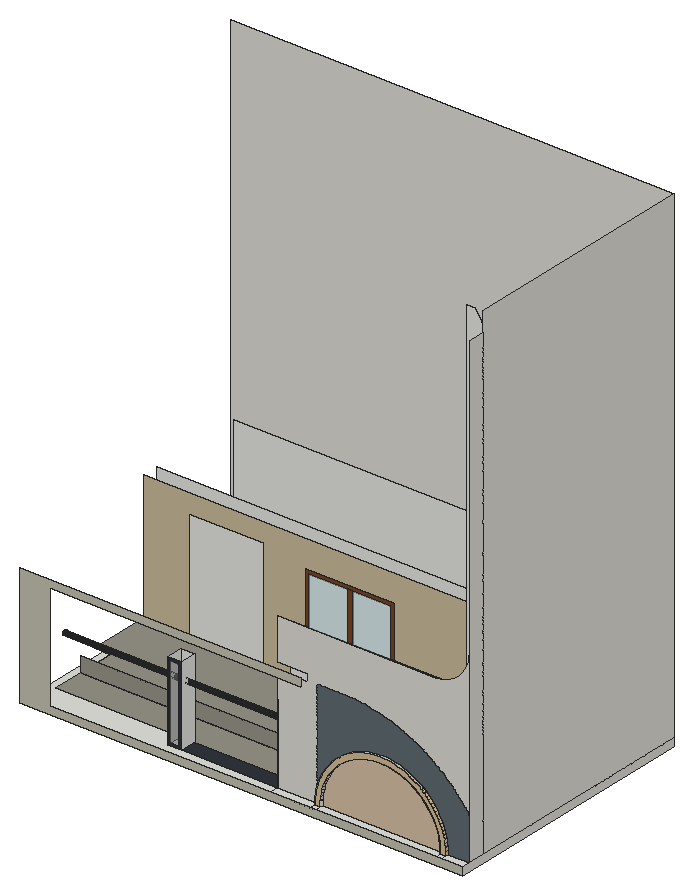
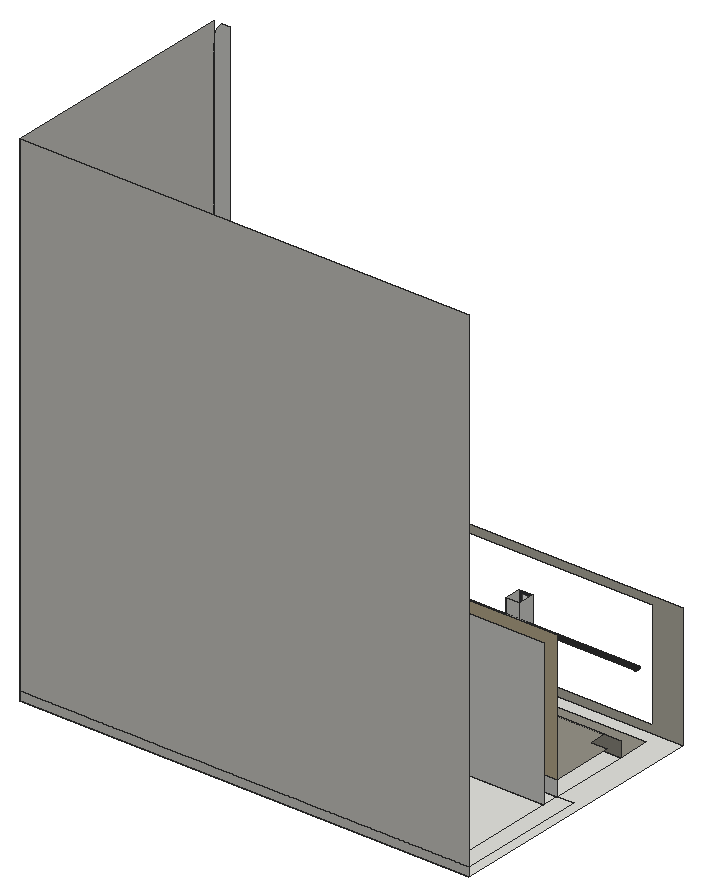
# SketchUp Ruby script. Lengths in inches.
U = 1.inch
M = Sketchup.active_model
def pt(a) = Geom::Point3d.new(a.map { |v| v * U })
def face(e, loops, mat)
  f = e.add_face(loops[0].map { |a| pt(a) })
  loops[1..].each { |l| e.add_face(l.map { |a| pt(a) }).erase! }
  f.material = f.back_material = mat if mat
  f
end
# faces: each face lists its corners as indices into pts; further lists are holes
def faces(e, pts, list, mat = nil) = list.each { |f| face(e, (f[0].is_a?(Array) ? f : [f]).map { |l| l.map { |i| pts[i] } }, mat) }
# xy, xz, yz: faces in a plane at the given z, y or x. An outline is a flat list of corners, or four numbers for a rectangle; further outlines are holes
def ring(l) = l.size == 4 ? [[l[0], l[1]], [l[2], l[1]], [l[2], l[3]], [l[0], l[3]]] : l.each_slice(2).to_a
def flat(e, list, mat, &to3) = list.each { |f| face(e, (f[0].is_a?(Array) ? f : [f]).map { |l| ring(l).map { |u, v| to3.(u, v) } }, mat) }
def xy(e, z, list, mat = nil) = flat(e, list, mat) { |x, y| [x, y, z] }
def xz(e, y, list, mat = nil) = flat(e, list, mat) { |x, z| [x, y, z] }
def yz(e, x, list, mat = nil) = flat(e, list, mat) { |y, z| [x, y, z] }
def lines(e, pts, list) = list.each { |a, b| e.add_line(pt(pts[a]), pt(pts[b])) }
# prism: a flat outline (further loops are holes) pulled along v
def prism(e, loops, v, mat = nil)
  f = face(e, loops, mat); d = Geom::Vector3d.new(v.map { |x| x * U })
  f.pushpull(f.normal.samedirection?(d) ? d.length : -d.length)
end
def box(e, o, s, mat = nil) = prism(e, [[o, [o[0] + s[0], o[1], o[2]], [o[0] + s[0], o[1] + s[1], o[2]], [o[0], o[1] + s[1], o[2]]]], [0, 0, s[2]], mat)
def at(x, y, z, deg = 0) = Geom::Transformation.translation(pt([x, y, z])) * Geom::Transformation.rotation(ORIGIN, Z_AXIS, deg.degrees)
def axes(o, x, y, z) = Geom::Transformation.new([*x, 0, *y, 0, *z, 0, *pt(o).to_a, 1])
def part(name) = M.definitions.add(name)
# library, detail: a bought-in or finely detailed component or shape, given as its bounding box
def library(name, o, s) = part(name).tap { |d| box(d.entities, o, s) }
def detail(e, o, s) = box(e.add_group.entities, o, s)
def put(e, d, t, mat = nil) = e.add_instance(d, t).tap { |i| i.material = mat if mat }
def group(e, t, mat = nil) = e.add_group.tap { |g| g.transformation = t; g.material = mat if mat }.entities
root = M.entities
M.materials.add("[Formica Beige]").color = [211, 187, 149]
M.materials.add("[Formica Graystone]").color = [193, 189, 175]
M.materials.add("[Formica Graystone]1").color = [149, 146, 135]
M.materials.add("[Formica Laminate Dark]").color = [50, 53, 60]
M.materials.add("[Formica Laminate Light]").color = [213, 189, 164]
M.materials.add("[Formica Speckled Grey]1").color = [94, 105, 111]
M.materials.add("[Quartz Light Brown]").color = [199, 184, 152]
M.materials.add("[Terrazzo Tile Light]").color = [219, 217, 210]
M.materials.add("[Translucent Glass Gray]").color = [128, 128, 128]
M.materials["[Translucent Glass Gray]"].alpha = 0.5
M.materials.add("[Translucent Glass Safety]").color = [204, 235, 244]
M.materials["[Translucent Glass Safety]"].alpha = 0.5
M.materials.add("[Wood Veneer 01]").color = [120, 70, 37]
xy(root,0,[[0,13.1875,490.375,305.18]])
xy(root,9,[[277.85,13.1875,321.38,22.75],[321.38,13.1875,327.45,19.625],[327.45,13.1875,460.44,22.75],[460.44,13.1875,466.51,19.625],[466.51,13.1875,490.375,22.75],
  [321.38,19.625,327.45,22.75],[460.44,19.625,466.51,22.75],[155.89,22.75,171.0625,40.6875],[277.85,22.75,490.375,40.6875],[472.4375,40.6875,490.375,162.27],
  [17.9375,75.25,472.4375,162.27],[0,162.27,0,305.18,490.375,305.18,490.375,162.27,472.4375,162.27,472.4375,287.24,17.9375,287.24,17.9375,162.27],[17.9375,162.27,472.4375,180.28],[17.9375,180.28,472.4375,287.24]])
xy(root,9,[[17.9375,40.6875,472.4375,75.25]],"[Formica Graystone]1")
xy(root,9,[[171.0625,22.75,277.85,40.6875]],"[Formica Laminate Dark]")
xy(root,25.4375,[[36.375,75.25,472.4375,75.25,472.4375,162.27,17.9375,162.27,17.9375,93.6875,36.375,93.6875]],"[Formica Graystone]1")
xz(root,13.1875,[[0,0,490.375,0,490.375,9,32.82,9,32.82,125.79,311.48,125.79,311.48,134.5,0,134.5]],"[Formica Graystone]")
xz(root,19.625,[[321.38,9,327.45,9,327.45,14.79,327.54,15.98,328,19.44,328.64,22.88,329.45,26.28,330.44,29.63,331.61,32.93,332.95,36.16,334.45,39.3125,336.12,42.38,337.95,45.36,339.93,48.25,342.06,51.02,344.33,53.68,346.73,56.21,349.27,58.62,351.93,60.89,354.7,63.02,357.58,65,360.5625,66.82,363.63,68.49,366.79,70,370.02,71.33,373.3125,72.5,376.66,73.49,380.0625,74.31,383.5,74.95,386.97,75.4,390.45,75.68,393.95,75.77,397.44,75.68,400.92,75.4,404.39,74.95,407.83,74.31,411.23,73.49,414.58,72.5,417.875,71.33,421.1,70,424.26,68.49,427.33,66.82,430.3125,65,433.19,63.02,435.96,60.89,438.62,58.62,441.16,56.21,443.56,53.68,445.83,51.02,447.96,48.25,449.94,45.36,451.77,42.38,453.4375,39.3125,454.94,36.16,456.28,32.93,457.45,29.63,458.4375,26.28,459.26,22.88,459.89,19.44,460.35,15.98,460.44,14.79,460.44,9,466.51,9,466.41,12.8,466.11,16.58,465.61,20.35,464.92,24.09,464.04,27.78,462.96,31.42,461.6875,35,460.23,38.51,458.6,41.94,456.79,45.28,454.8,48.52,452.65,51.65,450.34,54.67,447.87,57.55,445.26,60.31,442.5,62.92,439.61,65.39,436.6,67.7,433.47,69.86,430.23,71.84,426.89,73.65,423.46,75.29,419.95,76.74,416.37,78.01,412.73,79.09,409.03,79.98,405.3,80.67,401.53,81.16,397.74,81.46,393.95,81.5625,390.15,81.46,386.36,81.16,382.59,80.67,378.86,79.98,375.17,79.09,371.52,78.01,367.94,76.74,364.43,75.29,361,73.65,357.66,71.84,354.43,69.86,351.29,67.7,348.28,65.39,345.39,62.92,342.64,60.31,340.02,57.55,337.55,54.67,335.24,51.65,333.09,48.52,331.1,45.28,329.29,41.94,327.66,38.51,326.2,35,324.93,31.42,323.86,27.78,322.97,24.09,322.28,20.35,321.78,16.58,321.48,12.8]],"[Formica Beige]")
xz(root,22.75,[[321.38,9,321.48,12.8,321.78,16.58,322.28,20.35,322.97,24.09,323.86,27.78,324.93,31.42,326.2,35,327.66,38.51,329.29,41.94,331.1,45.28,333.09,48.52,335.24,51.65,337.55,54.67,340.02,57.55,342.64,60.31,345.39,62.92,348.28,65.39,351.29,67.7,354.43,69.86,357.66,71.84,361,73.65,364.43,75.29,367.94,76.74,371.52,78.01,375.17,79.09,378.86,79.98,382.59,80.67,386.36,81.16,390.15,81.46,393.95,81.5625,397.74,81.46,401.53,81.16,405.3,80.67,409.03,79.98,412.73,79.09,416.37,78.01,419.95,76.74,423.46,75.29,426.89,73.65,430.23,71.84,433.47,69.86,436.6,67.7,439.61,65.39,442.5,62.92,445.26,60.31,447.87,57.55,450.34,54.67,452.65,51.65,454.8,48.52,456.79,45.28,458.6,41.94,460.23,38.51,461.6875,35,462.96,31.42,464.04,27.78,464.92,24.09,465.61,20.35,466.11,16.58,466.41,12.8,466.51,9,460.44,9,460.44,14.79,460.35,15.98,459.89,19.44,459.26,22.88,458.4375,26.28,457.45,29.63,456.28,32.93,454.94,36.16,453.4375,39.3125,451.77,42.38,449.94,45.36,447.96,48.25,445.83,51.02,443.56,53.68,441.16,56.21,438.62,58.62,435.96,60.89,433.19,63.02,430.3125,65,427.33,66.82,424.26,68.49,421.1,70,417.875,71.33,414.58,72.5,411.23,73.49,407.83,74.31,404.39,74.95,400.92,75.4,397.44,75.68,393.95,75.77,390.45,75.68,386.97,75.4,383.5,74.95,380.0625,74.31,376.66,73.49,373.3125,72.5,370.02,71.33,366.79,70,363.63,68.49,360.5625,66.82,357.58,65,354.7,63.02,351.93,60.89,349.27,58.62,346.73,56.21,344.33,53.68,342.06,51.02,339.93,48.25,337.95,45.36,336.12,42.38,334.45,39.3125,332.95,36.16,331.61,32.93,330.44,29.63,329.45,26.28,328.64,22.88,328,19.44,327.54,15.98,327.45,14.79,327.45,9]])
xz(root,22.75,[[[155.89,9,171.0625,96.38],[158.36,11.46,168.6,93.92]]],"[Formica Laminate Dark]")
xz(root,22.75,[[327.45,9,460.44,9,460.44,14.79,460.35,15.98,459.89,19.44,459.26,22.88,458.4375,26.28,457.45,29.63,456.28,32.93,454.94,36.16,453.4375,39.3125,451.77,42.38,449.94,45.36,447.96,48.25,445.83,51.02,443.56,53.68,441.16,56.21,438.62,58.62,435.96,60.89,433.19,63.02,430.3125,65,427.33,66.82,424.26,68.49,421.1,70,417.875,71.33,414.58,72.5,411.23,73.49,407.83,74.31,404.39,74.95,400.92,75.4,397.44,75.68,393.95,75.77,390.45,75.68,386.97,75.4,383.5,74.95,380.0625,74.31,376.66,73.49,373.3125,72.5,370.02,71.33,366.79,70,363.63,68.49,360.5625,66.82,357.58,65,354.7,63.02,351.93,60.89,349.27,58.62,346.73,56.21,344.33,53.68,342.06,51.02,339.93,48.25,337.95,45.36,336.12,42.38,334.45,39.3125,332.95,36.16,331.61,32.93,330.44,29.63,329.45,26.28,328.64,22.88,328,19.44,327.54,15.98,327.45,14.79]],"[Formica Laminate Light]")
xz(root,22.75,[[321.38,9,321.48,12.8,321.78,16.58,322.28,20.35,322.97,24.09,323.86,27.78,324.93,31.42,326.2,35,327.66,38.51,329.29,41.94,331.1,45.28,333.09,48.52,335.24,51.65,337.55,54.67,340.02,57.55,342.64,60.31,345.39,62.92,348.28,65.39,351.29,67.7,354.43,69.86,357.66,71.84,361,73.65,364.43,75.29,367.94,76.74,371.52,78.01,375.17,79.09,378.86,79.98,382.59,80.67,386.36,81.16,390.15,81.46,393.95,81.5625,397.74,81.46,401.53,81.16,405.3,80.67,409.03,79.98,412.73,79.09,416.37,78.01,419.95,76.74,423.46,75.29,426.89,73.65,430.23,71.84,433.47,69.86,436.6,67.7,439.61,65.39,442.5,62.92,445.26,60.31,447.87,57.55,450.34,54.67,452.65,51.65,454.8,48.52,456.79,45.28,458.6,41.94,460.23,38.51,461.6875,35,462.96,31.42,464.04,27.78,464.92,24.09,465.61,20.35,466.11,16.58,466.41,12.8,466.51,9,490.375,9,490.375,56.28,488.74,58.47,487.08,60.63,485.375,62.77,483.64,64.875,481.875,66.96,480.08,69.01,478.25,71.04,476.38,73.03,474.49,75,472.57,76.9375,470.61,78.85,468.63,80.72,466.62,82.57,464.58,84.38,462.51,86.16,460.41,87.91,458.29,89.63,456.14,91.31,453.96,92.96,451.76,94.57,449.53,96.15,447.28,97.7,445.01,99.21,442.71,100.68,440.39,102.12,438.04,103.52,435.68,104.89,433.29,106.21,430.89,107.5,428.46,108.76,426.02,109.97,423.55,111.15,421.07,112.28,418.57,113.38,416.05,114.44,413.52,115.46,410.97,116.44,408.41,117.38,405.83,118.28,403.24,119.14,400.64,119.96,398.02,120.74,395.39,121.48,392.75,122.17,390.1,122.83,387.4375,123.44,384.77,124.01,382.09,124.54,379.4,125.03,376.71,125.48,374.01,125.88,371.3,126.24,368.59,126.5625,365.875,126.84,363.16,127.07,360.43,127.26,357.71,127.41,354.98,127.52,352.25,127.58,349.52,127.6,321.38,127.6]],"[Formica Speckled Grey]1")
xz(root,22.75,[[277.85,9,321.38,9,321.38,127.6,349.52,127.6,352.25,127.58,354.98,127.52,357.71,127.41,360.43,127.26,363.16,127.07,365.875,126.84,368.59,126.5625,371.3,126.24,374.01,125.88,376.71,125.48,379.4,125.03,382.09,124.54,384.77,124.01,387.4375,123.44,390.1,122.83,392.75,122.17,395.39,121.48,398.02,120.74,400.64,119.96,403.24,119.14,405.83,118.28,408.41,117.38,410.97,116.44,413.52,115.46,416.05,114.44,418.57,113.38,421.07,112.28,423.55,111.15,426.02,109.97,428.46,108.76,430.89,107.5,433.29,106.21,435.68,104.89,438.04,103.52,440.39,102.12,442.71,100.68,445.01,99.21,447.28,97.7,449.53,96.15,451.76,94.57,453.96,92.96,456.14,91.31,458.29,89.63,460.41,87.91,462.51,86.16,464.58,84.38,466.62,82.57,468.63,80.72,470.61,78.85,472.57,76.9375,474.49,75,476.38,73.03,478.25,71.04,480.08,69.01,481.875,66.96,483.64,64.875,485.375,62.77,487.08,60.63,488.74,58.47,490.375,56.28,490.375,218.09,490.05,213.06,489.0625,208.12,487.44,203.35,485.21,198.83,482.41,194.64,479.09,190.85,475.3,187.52,471.11,184.72,466.59,182.5,461.82,180.875,456.88,179.89,451.85,179.5625,277.85,179.5625,277.85,134.5,311.48,134.5,311.48,125.79,277.85,125.79]],"[Terrazzo Tile Light]")
xz(root,22.75,[[158.36,11.46,168.6,93.92]],"[Translucent Glass Gray]")
xz(root,40.6875,[[155.89,9,171.0625,96.38],[277.85,9,472.4375,167.375],[472.4375,9,490.375,9,490.375,527.88,490.12,531.85,489.34,535.76,488.06,539.53,486.3,543.1,484.09,546.41,481.46,549.4,481.42,549.4375,472.4375,549.4375]])
xz(root,75.25,[[17.9375,9,472.4375,25.4375]],"[Formica Graystone]1")
xz(root,162.27,[[17.9375,9,472.4375,25.4375]])
xz(root,162.27,[[[17.9375,25.4375,67.875,25.4375,67.875,146.5,151.125,146.5,151.125,25.4375,472.4375,25.4375,472.4375,167.375,17.9375,167.375],[196.22,54.31,296.22,137.43]]],"[Quartz Light Brown]")
xz(root,162.27,[[200.64,58.73,243.71,133.01],[249.21,58.73,291.8,133.01]],"[Translucent Glass Safety]")
xz(root,162.27,[[[196.22,54.31,296.22,137.43],[200.64,58.73,291.8,133.01]],[243.71,58.73,249.21,133.01]],"[Wood Veneer 01]")
xz(root,180.28,[[17.9375,9,472.4375,167.375]])
xz(root,287.24,[[17.9375,9,472.4375,167.375]])
xz(root,305.18,[[0,0,490.375,9],[0,9,490.375,549.4375]],"[Terrazzo Tile Light]")
yz(root,155.89,[[22.75,9,40.6875,96.38]])
yz(root,171.0625,[[22.75,9,40.6875,96.38]])
yz(root,277.85,[[33.12,13.1,33.67,13.17,34.18,13.39,34.62,13.72,34.96,14.16,35.17,14.68,35.24,15.23,35.17,15.78,34.96,16.29,34.62,16.73,34.18,17.07,33.67,17.28,33.12,17.35,32.57,17.28,32.05,17.07,31.61,16.73,31.28,16.29,31.06,15.78,30.99,15.23,31.06,14.68,31.28,14.16,31.61,13.72,32.05,13.39,32.57,13.17],[33.12,21.91,33.67,21.99,34.18,22.2,34.62,22.54,34.96,22.98,35.17,23.49,35.24,24.04,35.17,24.59,34.96,25.1,34.62,25.54,34.18,25.88,33.67,26.09,33.12,26.16,32.57,26.09,32.05,25.88,31.61,25.54,31.28,25.1,31.06,24.59,30.99,24.04,31.06,23.49,31.28,22.98,31.61,22.54,32.05,22.2,32.57,21.99],[33.12,32.23,33.67,32.3,34.18,32.51,34.62,32.85,34.96,33.29,35.17,33.8,35.24,34.35,35.17,34.9,34.96,35.41,34.62,35.85,34.18,36.19,33.67,36.4,33.12,36.48,32.57,36.4,32.05,36.19,31.61,35.85,31.28,35.41,31.06,34.9,30.99,34.35,31.06,33.8,31.28,33.29,31.61,32.85,32.05,32.51,32.57,32.3],[33.12,41.23,33.67,41.3,34.18,41.51,34.62,41.85,34.96,42.29,35.17,42.8,35.24,43.35,35.17,43.9,34.96,44.41,34.62,44.85,34.18,45.19,33.67,45.4,33.12,45.48,32.57,45.4,32.05,45.19,31.61,44.85,31.28,44.41,31.06,43.9,30.99,43.35,31.06,42.8,31.28,42.29,31.61,41.85,32.05,41.51,32.57,41.3],[33.12,50.23,33.67,50.3,34.18,50.51,34.62,50.85,34.96,51.29,35.17,51.8,35.24,52.35,35.17,52.9,34.96,53.41,34.62,53.85,34.18,54.19,33.67,54.4,33.12,54.48,32.57,54.4,32.05,54.19,31.61,53.85,31.28,53.41,31.06,52.9,30.99,52.35,31.06,51.8,31.28,51.29,31.61,50.85,32.05,50.51,32.57,50.3],
  [33.12,60.04,33.67,60.11,34.18,60.32,34.62,60.66,34.96,61.1,35.17,61.61,35.24,62.16,35.17,62.71,34.96,63.23,34.62,63.67,34.18,64,33.67,64.22,33.12,64.29,32.57,64.22,32.05,64,31.61,63.67,31.28,63.23,31.06,62.71,30.99,62.16,31.06,61.61,31.28,61.1,31.61,60.66,32.05,60.32,32.57,60.11],[33.12,70.48,33.67,70.55,34.18,70.76,34.62,71.1,34.96,71.54,35.17,72.05,35.24,72.6,35.17,73.15,34.96,73.66,34.62,74.1,34.18,74.44,33.67,74.65,33.12,74.73,32.57,74.65,32.05,74.44,31.61,74.1,31.28,73.66,31.06,73.15,30.99,72.6,31.06,72.05,31.28,71.54,31.61,71.1,32.05,70.76,32.57,70.55]])
yz(root,277.85,[[[22.75,9,40.6875,96.38],[33.12,13.1,33.67,13.17,34.18,13.39,34.62,13.72,34.96,14.16,35.17,14.68,35.24,15.23,35.17,15.78,34.96,16.29,34.62,16.73,34.18,17.07,33.67,17.28,33.12,17.35,32.57,17.28,32.05,17.07,31.61,16.73,31.28,16.29,31.06,15.78,30.99,15.23,31.06,14.68,31.28,14.16,31.61,13.72,32.05,13.39,32.57,13.17],[33.12,80.16,33.67,80.24,34.18,80.45,34.62,80.79,34.96,81.23,35.17,81.74,35.24,82.29,35.17,82.84,34.96,83.35,34.62,83.79,34.18,84.13,33.67,84.34,33.12,84.41,32.57,84.34,32.05,84.13,31.61,83.79,31.28,83.35,31.06,82.84,30.99,82.29,31.06,81.74,31.28,81.23,31.61,80.79,32.05,80.45,32.57,80.24],[33.12,21.91,33.67,21.99,34.18,22.2,34.62,22.54,34.96,22.98,35.17,23.49,35.24,24.04,35.17,24.59,34.96,25.1,34.62,25.54,34.18,25.88,33.67,26.09,33.12,26.16,32.57,26.09,32.05,25.88,31.61,25.54,31.28,25.1,31.06,24.59,30.99,24.04,31.06,23.49,31.28,22.98,31.61,22.54,32.05,22.2,32.57,21.99],[33.12,70.48,33.67,70.55,34.18,70.76,34.62,71.1,34.96,71.54,35.17,72.05,35.24,72.6,35.17,73.15,34.96,73.66,34.62,74.1,34.18,74.44,33.67,74.65,33.12,74.73,32.57,74.65,32.05,74.44,31.61,74.1,31.28,73.66,31.06,73.15,30.99,72.6,31.06,72.05,31.28,71.54,31.61,71.1,32.05,70.76,32.57,70.55],[33.12,32.23,33.67,32.3,34.18,32.51,34.62,32.85,34.96,33.29,35.17,33.8,35.24,34.35,35.17,34.9,34.96,35.41,34.62,35.85,34.18,36.19,33.67,36.4,33.12,36.48,32.57,36.4,32.05,36.19,31.61,35.85,31.28,35.41,31.06,34.9,30.99,34.35,31.06,33.8,31.28,33.29,31.61,32.85,32.05,32.51,32.57,32.3],[33.12,60.04,33.67,60.11,34.18,60.32,34.62,60.66,34.96,61.1,35.17,61.61,35.24,62.16,35.17,62.71,34.96,63.23,34.62,63.67,34.18,64,33.67,64.22,33.12,64.29,32.57,64.22,32.05,64,31.61,63.67,31.28,63.23,31.06,62.71,30.99,62.16,31.06,61.61,31.28,61.1,31.61,60.66,32.05,60.32,32.57,60.11],[33.12,88.66,33.67,88.74,34.18,88.95,34.62,89.29,34.96,89.73,35.17,90.24,35.24,90.79,35.17,91.34,34.96,91.85,34.62,92.29,34.18,92.63,33.67,92.84,33.12,92.91,32.57,92.84,32.05,92.63,31.61,92.29,31.28,91.85,31.06,91.34,30.99,90.79,31.06,90.24,31.28,89.73,31.61,89.29,32.05,88.95,32.57,88.74],[33.12,41.23,33.67,41.3,34.18,41.51,34.62,41.85,34.96,42.29,35.17,42.8,35.24,43.35,35.17,43.9,34.96,44.41,34.62,44.85,34.18,45.19,33.67,45.4,33.12,45.48,32.57,45.4,32.05,45.19,31.61,44.85,31.28,44.41,31.06,43.9,30.99,43.35,31.06,42.8,31.28,42.29,31.61,41.85,32.05,41.51,32.57,41.3],[33.12,50.23,33.67,50.3,34.18,50.51,34.62,50.85,34.96,51.29,35.17,51.8,35.24,52.35,35.17,52.9,34.96,53.41,34.62,53.85,34.18,54.19,33.67,54.4,33.12,54.48,32.57,54.4,32.05,54.19,31.61,53.85,31.28,53.41,31.06,52.9,30.99,52.35,31.06,51.8,31.28,51.29,31.61,50.85,32.05,50.51,32.57,50.3]]],"[Formica Graystone]1")
yz(root,327.45,[[19.625,9,22.75,14.79]])
yz(root,460.44,[[19.625,9,22.75,14.79]])
yz(root,472.4375,[[75.25,9,162.27,25.4375],[162.27,9,180.28,167.375],[180.28,9,287.24,167.375]])
yz(root,472.4375,[[40.6875,9,75.25,167.375],[75.25,25.4375,162.27,167.375]],"[Quartz Light Brown]")
yz(root,490.375,[[13.1875,0,305.18,9],[22.75,9,40.6875,527.88],[40.6875,9,305.18,549.4375]],"[Terrazzo Tile Light]")
p = [[321.48,22.75,12.8],[321.38,22.75,9],[321.38,19.625,9],[321.48,19.625,12.8],[466.51,22.75,9],[466.41,22.75,12.8],
  [466.41,19.625,12.8],[466.51,19.625,9],[321.78,22.75,16.58],[321.78,19.625,16.58],[466.11,22.75,16.58],[466.11,19.625,16.58],
  [327.45,22.75,14.79],[327.54,22.75,15.98],[327.54,19.625,15.98],[327.45,19.625,14.79],[460.35,22.75,15.98],[460.44,22.75,14.79],
  [460.44,19.625,14.79],[460.35,19.625,15.98],[328,22.75,19.44],[328,19.625,19.44],[459.89,22.75,19.44],[459.89,19.625,19.44],
  [322.28,22.75,20.35],[322.28,19.625,20.35],[465.61,22.75,20.35],[465.61,19.625,20.35],[328.64,22.75,22.88],[328.64,19.625,22.88],
  [459.26,22.75,22.88],[459.26,19.625,22.88],[322.97,22.75,24.09],[322.97,19.625,24.09],[464.92,22.75,24.09],[464.92,19.625,24.09],
  [329.45,22.75,26.28],[329.45,19.625,26.28],[458.4375,22.75,26.28],[458.4375,19.625,26.28],[323.86,22.75,27.78],[323.86,19.625,27.78],
  [464.04,22.75,27.78],[464.04,19.625,27.78],[330.44,22.75,29.63],[330.44,19.625,29.63],[457.45,22.75,29.63],[457.45,19.625,29.63],
  [324.93,22.75,31.42],[324.93,19.625,31.42],[462.96,22.75,31.42],[462.96,19.625,31.42],[331.61,22.75,32.93],[331.61,19.625,32.93],
  [456.28,22.75,32.93],[456.28,19.625,32.93],[326.2,22.75,35],[326.2,19.625,35],[461.6875,22.75,35],[461.6875,19.625,35],
  [332.95,22.75,36.16],[332.95,19.625,36.16],[454.94,22.75,36.16],[454.94,19.625,36.16],[327.66,22.75,38.51],[327.66,19.625,38.51],
  [460.23,22.75,38.51],[460.23,19.625,38.51],[334.45,22.75,39.3125],[334.45,19.625,39.3125],[453.4375,22.75,39.3125],[453.4375,19.625,39.3125],
  [329.29,22.75,41.94],[329.29,19.625,41.94],[458.6,22.75,41.94],[458.6,19.625,41.94],[336.12,22.75,42.38],[336.12,19.625,42.38],
  [451.77,22.75,42.38],[451.77,19.625,42.38],[331.1,22.75,45.28],[331.1,19.625,45.28],[456.79,22.75,45.28],[456.79,19.625,45.28],
  [337.95,22.75,45.36],[337.95,19.625,45.36],[449.94,22.75,45.36],[449.94,19.625,45.36],[333.09,22.75,48.52],[333.09,19.625,48.52],
  [454.8,22.75,48.52],[454.8,19.625,48.52],[339.93,22.75,48.25],[339.93,19.625,48.25],[447.96,22.75,48.25],[447.96,19.625,48.25],
  [342.06,22.75,51.02],[342.06,19.625,51.02],[445.83,22.75,51.02],[445.83,19.625,51.02],[335.24,22.75,51.65],[335.24,19.625,51.65],
  [452.65,22.75,51.65],[452.65,19.625,51.65],[344.33,22.75,53.68],[344.33,19.625,53.68],[443.56,22.75,53.68],[443.56,19.625,53.68],
  [337.55,22.75,54.67],[337.55,19.625,54.67],[450.34,22.75,54.67],[450.34,19.625,54.67],[346.73,22.75,56.21],[346.73,19.625,56.21],
  [441.16,22.75,56.21],[441.16,19.625,56.21],[340.02,22.75,57.55],[340.02,19.625,57.55],[447.87,22.75,57.55],[447.87,19.625,57.55],
  [349.27,22.75,58.62],[349.27,19.625,58.62],[438.62,22.75,58.62],[438.62,19.625,58.62],[342.64,22.75,60.31],[342.64,19.625,60.31],
  [445.26,22.75,60.31],[445.26,19.625,60.31],[351.93,22.75,60.89],[351.93,19.625,60.89],[435.96,22.75,60.89],[435.96,19.625,60.89],
  [345.39,22.75,62.92],[345.39,19.625,62.92],[442.5,22.75,62.92],[442.5,19.625,62.92],[354.7,22.75,63.02],[354.7,19.625,63.02],
  [433.19,22.75,63.02],[433.19,19.625,63.02],[348.28,22.75,65.39],[348.28,19.625,65.39],[439.61,22.75,65.39],[439.61,19.625,65.39],
  [357.58,22.75,65],[357.58,19.625,65],[430.3125,22.75,65],[430.3125,19.625,65],[360.5625,22.75,66.82],[360.5625,19.625,66.82],
  [427.33,22.75,66.82],[427.33,19.625,66.82],[351.29,22.75,67.7],[351.29,19.625,67.7],[436.6,22.75,67.7],[436.6,19.625,67.7],
  [363.63,22.75,68.49],[363.63,19.625,68.49],[424.26,22.75,68.49],[424.26,19.625,68.49],[354.43,22.75,69.86],[354.43,19.625,69.86],
  [433.47,22.75,69.86],[433.47,19.625,69.86],[366.79,22.75,70],[366.79,19.625,70],[421.1,22.75,70],[421.1,19.625,70],
  [357.66,22.75,71.84],[357.66,19.625,71.84],[430.23,22.75,71.84],[430.23,19.625,71.84],[370.02,22.75,71.33],[370.02,19.625,71.33],
  [417.875,22.75,71.33],[417.875,19.625,71.33],[277.85,32.05,70.76],[277.85,31.61,71.1],[32.82,31.61,71.1],[32.82,32.05,70.76],
  [277.85,34.62,71.1],[277.85,34.18,70.76],[32.82,34.18,70.76],[32.82,34.62,71.1],[277.85,31.28,71.54],[32.82,31.28,71.54],
  [277.85,34.96,71.54],[32.82,34.96,71.54],[373.3125,22.75,72.5],[373.3125,19.625,72.5],[414.58,22.75,72.5],[414.58,19.625,72.5],
  [277.85,31.06,72.05],[32.82,31.06,72.05],[277.85,35.17,72.05],[32.82,35.17,72.05],[361,22.75,73.65],[361,19.625,73.65],
  [426.89,22.75,73.65],[426.89,19.625,73.65],[277.85,30.99,72.6],[32.82,30.99,72.6],[277.85,35.24,72.6],[32.82,35.24,72.6],
  [376.66,22.75,73.49],[376.66,19.625,73.49],[411.23,22.75,73.49],[411.23,19.625,73.49],[277.85,31.06,73.15],[32.82,31.06,73.15],
  [277.85,35.17,73.15],[32.82,35.17,73.15],[277.85,31.28,73.66],[32.82,31.28,73.66],[277.85,34.96,73.66],[32.82,34.96,73.66],
  [380.0625,22.75,74.31],[380.0625,19.625,74.31],[407.83,22.75,74.31],[407.83,19.625,74.31],[364.43,22.75,75.29],[364.43,19.625,75.29],
  [423.46,22.75,75.29],[423.46,19.625,75.29],[277.85,31.61,74.1],[32.82,31.61,74.1],[277.85,34.62,74.1],[32.82,34.62,74.1],
  [277.85,32.05,74.44],[32.82,32.05,74.44],[277.85,34.18,74.44],[32.82,34.18,74.44],[383.5,22.75,74.95],[383.5,19.625,74.95],
  [404.39,22.75,74.95],[404.39,19.625,74.95],[277.85,32.57,74.65],[32.82,32.57,74.65],[277.85,33.67,74.65],[32.82,33.67,74.65],
  [277.85,33.12,74.73],[32.82,33.12,74.73],[386.97,22.75,75.4],[386.97,19.625,75.4],[400.92,22.75,75.4],[400.92,19.625,75.4],
  [367.94,22.75,76.74],[367.94,19.625,76.74],[419.95,22.75,76.74],[419.95,19.625,76.74],[390.45,22.75,75.68],[390.45,19.625,75.68],
  [397.44,22.75,75.68],[397.44,19.625,75.68],[393.95,22.75,75.77],[393.95,19.625,75.77]]
faces(root,p,[[0,1,2,3],[4,5,6,7],[8,0,3,9],[5,10,11,6],[24,8,9,25],[10,26,27,11],[32,24,25,33],[26,34,35,27],
  [40,32,33,41],[34,42,43,35],[48,40,41,49],[42,50,51,43],[56,48,49,57],[50,58,59,51],[64,56,57,65],[58,66,67,59],
  [72,64,65,73],[66,74,75,67],[80,72,73,81],[74,82,83,75],[88,80,81,89],[82,90,91,83],[100,88,89,101],[90,102,103,91],
  [108,100,101,109],[102,110,111,103],[116,108,109,117],[110,118,119,111],[124,116,117,125],[118,126,127,119],[132,124,125,133],[126,134,135,127],
  [140,132,133,141],[134,142,143,135],[152,140,141,153],[142,154,155,143],[160,152,153,161],[154,162,163,155],[168,160,161,169],[162,170,171,163],
  [196,168,169,197],[170,198,199,171],[220,196,197,221],[198,222,223,199],[246,220,221,247],[222,248,249,223]],"[Formica Beige]")
faces(root,p,[[12,13,14,15],[16,17,18,19],[13,20,21,14],[22,16,19,23],[20,28,29,21],[30,22,23,31],[28,36,37,29],[38,30,31,39],
  [36,44,45,37],[46,38,39,47],[44,52,53,45],[54,46,47,55],[52,60,61,53],[62,54,55,63],[60,68,69,61],[70,62,63,71],
  [68,76,77,69],[78,70,71,79],[76,84,85,77],[86,78,79,87],[84,92,93,85],[94,86,87,95],[92,96,97,93],[98,94,95,99],
  [96,104,105,97],[106,98,99,107],[104,112,113,105],[114,106,107,115],[112,120,121,113],[122,114,115,123],[120,128,129,121],[130,122,123,131],
  [128,136,137,129],[138,130,131,139],[136,144,145,137],[146,138,139,147],[144,148,149,145],[150,146,147,151],[148,156,157,149],[158,150,151,159],
  [156,164,165,157],[166,158,159,167],[164,172,173,165],[174,166,167,175],[172,188,189,173],[190,174,175,191],[188,204,205,189],[206,190,191,207],
  [204,216,217,205],[218,206,207,219],[216,232,233,217],[234,218,219,235],[232,242,243,233],[244,234,235,245],[242,250,251,243],[252,244,245,253],
  [250,254,255,251],[254,252,253,255]])
faces(root,p,[[176,177,178,179],[180,181,182,183],[177,184,185,178],[186,180,183,187],[184,192,193,185],[194,186,187,195],[192,200,201,193],[202,194,195,203],
  [200,208,209,201],[210,202,203,211],[208,212,213,209],[214,210,211,215],[212,224,225,213],[226,214,215,227],[224,228,229,225],[230,226,227,231],
  [228,236,237,229],[238,230,231,239],[236,240,241,237],[240,238,239,241]],"[Formica Laminate Dark]")
